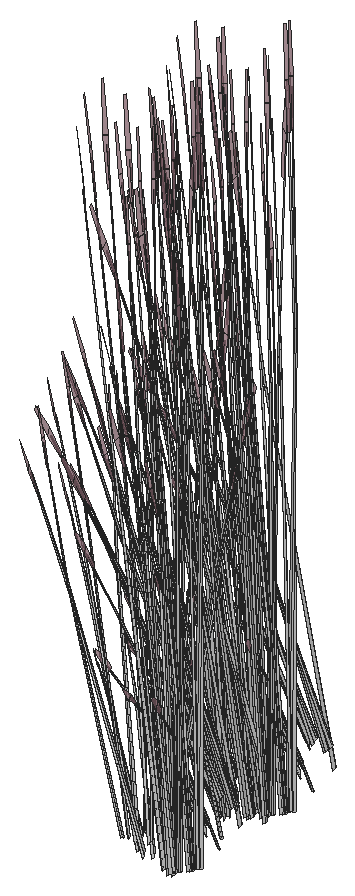
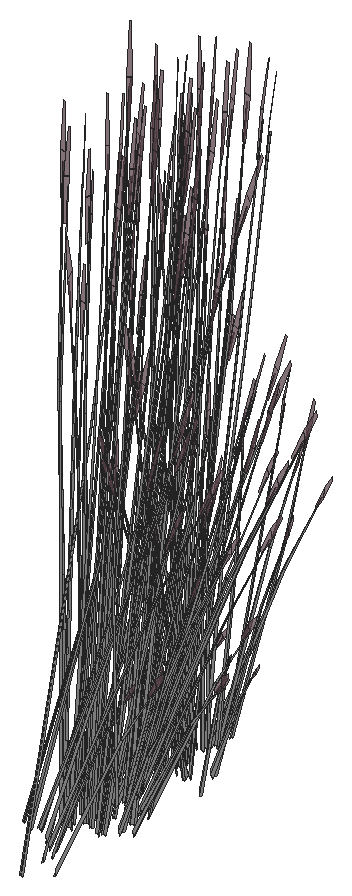
# SketchUp Ruby script. Lengths in inches.
U = 1.inch
M = Sketchup.active_model
def pt(a) = Geom::Point3d.new(a.map { |v| v * U })
def face(e, loops, mat)
  f = e.add_face(loops[0].map { |a| pt(a) })
  loops[1..].each { |l| e.add_face(l.map { |a| pt(a) }).erase! }
  f.material = f.back_material = mat if mat
  f
end
# faces: each face lists its corners as indices into pts; further lists are holes
def faces(e, pts, list, mat = nil) = list.each { |f| face(e, (f[0].is_a?(Array) ? f : [f]).map { |l| l.map { |i| pts[i] } }, mat) }
# xy, xz, yz: faces in a plane at the given z, y or x. An outline is a flat list of corners, or four numbers for a rectangle; further outlines are holes
def ring(l) = l.size == 4 ? [[l[0], l[1]], [l[2], l[1]], [l[2], l[3]], [l[0], l[3]]] : l.each_slice(2).to_a
def flat(e, list, mat, &to3) = list.each { |f| face(e, (f[0].is_a?(Array) ? f : [f]).map { |l| ring(l).map { |u, v| to3.(u, v) } }, mat) }
def xy(e, z, list, mat = nil) = flat(e, list, mat) { |x, y| [x, y, z] }
def xz(e, y, list, mat = nil) = flat(e, list, mat) { |x, z| [x, y, z] }
def yz(e, x, list, mat = nil) = flat(e, list, mat) { |y, z| [x, y, z] }
def lines(e, pts, list) = list.each { |a, b| e.add_line(pt(pts[a]), pt(pts[b])) }
# prism: a flat outline (further loops are holes) pulled along v
def prism(e, loops, v, mat = nil)
  f = face(e, loops, mat); d = Geom::Vector3d.new(v.map { |x| x * U })
  f.pushpull(f.normal.samedirection?(d) ? d.length : -d.length)
end
def box(e, o, s, mat = nil) = prism(e, [[o, [o[0] + s[0], o[1], o[2]], [o[0] + s[0], o[1] + s[1], o[2]], [o[0], o[1] + s[1], o[2]]]], [0, 0, s[2]], mat)
def at(x, y, z, deg = 0) = Geom::Transformation.translation(pt([x, y, z])) * Geom::Transformation.rotation(ORIGIN, Z_AXIS, deg.degrees)
def axes(o, x, y, z) = Geom::Transformation.new([*x, 0, *y, 0, *z, 0, *pt(o).to_a, 1])
def part(name) = M.definitions.add(name)
# library, detail: a bought-in or finely detailed component or shape, given as its bounding box
def library(name, o, s) = part(name).tap { |d| box(d.entities, o, s) }
def detail(e, o, s) = box(e.add_group.entities, o, s)
def put(e, d, t, mat = nil) = e.add_instance(d, t).tap { |i| i.material = mat if mat }
def group(e, t, mat = nil) = e.add_group.tap { |g| g.transformation = t; g.material = mat if mat }.entities
root = M.entities
M.materials.add("LightPink_Translucent").color = [144, 107, 117]
M.materials["LightPink_Translucent"].alpha = 0.75
M.materials.add("[_0053_Ivory_]").color = [200, 200, 200]
c1 = part("blade")
p = [[2.15,0.21,22],[0,0.17,0],[0.09,0.45,0],[2.18,0.31,22],[2.29,0.31,22],[0.38,0.45,0],
  [2.48,0.24,33],[2.49,0.24,33],[2.48,0.22,33]]
faces(c1.entities,p,[[0,1,2,3],[4,5,2,3],[6,3,4,7],[8,0,3,6]])
c2 = part("seeds")
p = [[0.3,-0.1,1.38],[-0.01,-0.03,1.59],[-0.01,-0.03,0.03],[0.14,-0.07,-0.07],[0.29,-0.03,3],[0.15,0.01,3.11]]
faces(c2.entities,p,[[0,1,2,3],[1,0,4,5]],"LightPink_Translucent")
c3 = part("blade with seeds")
put(c3.entities,c1,at(0,0,0))
put(c3.entities,c2,axes([2.4,0.25,30.99],[1.5799,-0.05474,1.17369],[-0.12525,1.92788,0.29478],[-0.07173,-0.02425,1.56792]))
put(root,c3,axes([629.08,303.62,255.53],[0.25192,-0.01424,1.71376],[-0.16712,0.61729,0.13857],[-0.35901,-0.03818,0.73262]),"[_0053_Ivory_]")
put(root,c3,axes([629.1875,294.41,255.53],[0.21074,-0.13302,1.71376],[0.17741,0.61464,0.13857],[-0.33083,0.13891,0.73262]),"[_0053_Ivory_]")
put(root,c3,axes([629.1875,304.71,255.53],[0.21074,-0.13302,1.71376],[0.17741,0.61464,0.13857],[-0.33083,0.13891,0.73262]),"[_0053_Ivory_]")
put(root,c3,axes([628.53,295.46,254.24],[0.21107,0.05162,1.43002],[0.13604,0.52729,-0.30754],[-0.28671,0.0987,0.61141]),"[_0053_Ivory_]")
put(root,c3,axes([628.53,305.75,254.24],[0.21107,0.05162,1.43002],[0.13604,0.52729,-0.30754],[-0.28671,0.0987,0.61141]),"[_0053_Ivory_]")
put(root,c3,axes([630.4,293.77,255],[0.17264,-0.09097,1.77064],[0.05953,0.63516,0.13857],[-0.37394,0.08428,0.63284]),"[_0053_Ivory_]")
put(root,c3,axes([630.4,304.0625,255],[0.17264,-0.09097,1.77064],[0.05953,0.63516,0.13857],[-0.37394,0.08428,0.63284]),"[_0053_Ivory_]")
put(root,c3,axes([629.83,303.05,256.63],[-0.60713,-0.01514,-0.71045],[0.04078,-0.63759,0.08574],[-0.25721,-0.06729,1.00501]),"[_0053_Ivory_]")
put(root,c3,axes([629.35,303.2,254.24],[0.11858,0.17508,1.43002],[-0.27325,0.4759,-0.30754],[-0.28057,-0.11375,0.61141]),"[_0053_Ivory_]")
put(root,c3,axes([628.86,293.85,256.18],[-0.50475,-0.17543,-0.35414],[0.14722,-0.5118,0.4572],[-0.20322,0.04693,0.87481]),"[_0053_Ivory_]")
put(root,c3,axes([628.86,304.15,256.18],[-0.50475,-0.17543,-0.35414],[0.14722,-0.5118,0.4572],[-0.20322,0.04693,0.87481]),"[_0053_Ivory_]")
put(root,c3,axes([629.56,302.63,255.53],[0.2256,0.10835,1.71376],[-0.46687,0.45453,0.13857],[-0.29098,-0.20505,0.73262]),"[_0053_Ivory_]")
put(root,c3,axes([629.56,313.02,255.53],[0.2256,0.10835,1.71376],[-0.46687,0.45453,0.13857],[-0.29098,-0.20505,0.73262]),"[_0053_Ivory_]")
put(root,c3,axes([629.21,294.12,256.33],[-0.16454,0.57202,-0.51099],[-0.56413,-0.19607,-0.3958],[-0.22713,0.05245,0.97773]),"[_0053_Ivory_]")
put(root,c3,axes([629.21,304.41,256.33],[-0.16454,0.57202,-0.51099],[-0.56413,-0.19607,-0.3958],[-0.22713,0.05245,0.97773]),"[_0053_Ivory_]")
put(root,c3,axes([629.63,303.17,256.33],[-0.44101,0.41656,-0.51099],[-0.38623,-0.44004,-0.3958],[-0.22407,-0.06338,0.97773]),"[_0053_Ivory_]")
put(root,c3,axes([628.92,304.375,253.15],[0.0154,0.09911,1.76342],[-0.31051,0.51756,-0.26939],[-0.22056,-0.02609,0.30037]),"[_0053_Ivory_]")
put(root,c3,axes([628.09,296.5625,254.42],[0.25312,-0.28501,1.1486],[0.09988,0.45119,0.84392],[-0.18292,0.08079,0.25299]),"[_0053_Ivory_]")
put(root,c3,axes([628.09,306.86,254.42],[0.25312,-0.28501,1.1486],[0.09988,0.45119,0.84392],[-0.18292,0.08079,0.25299]),"[_0053_Ivory_]")
put(root,c3,axes([629.47,302.78,256.18],[-0.34557,-0.39372,-0.35414],[0.39459,-0.37271,0.4572],[-0.20048,-0.05671,0.87481]),"[_0053_Ivory_]")
put(root,c3,axes([629.96,294.82,255.53],[0.1517,-0.19322,1.71376],[0.38303,0.52154,0.13857],[-0.26271,0.23751,0.73262]),"[_0053_Ivory_]")
put(root,c3,axes([629.96,305.12,255.53],[0.1517,-0.19322,1.71376],[0.38303,0.52154,0.13857],[-0.26271,0.23751,0.73262]),"[_0053_Ivory_]")
put(root,c3,axes([629.04,295.33,256.18],[-0.52868,0.08987,-0.35414],[-0.1396,-0.51376,0.4572],[-0.1515,0.13799,0.87481]),"[_0053_Ivory_]")
put(root,c3,axes([629.04,305.625,256.18],[-0.52868,0.08987,-0.35414],[-0.1396,-0.51376,0.4572],[-0.1515,0.13799,0.87481]),"[_0053_Ivory_]")
put(root,c3,axes([628.76,296.86,253.15],[0.08147,0.06283,1.76342],[0.13814,0.58211,-0.26939],[-0.18056,0.12413,0.30037]),"[_0053_Ivory_]")
put(root,c3,axes([628.64,303.73,254.42],[0.38775,-0.045,1.1486],[-0.24596,0.39648,0.84392],[-0.19161,-0.05948,0.25299]),"[_0053_Ivory_]")
put(root,c3,axes([629.84,295.3,255.53],[0.11309,-0.21615,1.71376],[0.47441,0.44731,0.13857],[-0.21402,0.27879,0.73262]),"[_0053_Ivory_]")
put(root,c3,axes([629.48,295.39,256.33],[0.15602,0.5742,-0.51099],[-0.59087,0.10045,-0.3958],[-0.16933,0.15423,0.97773]),"[_0053_Ivory_]")
put(root,c3,axes([629.48,305.69,256.33],[0.15602,0.5742,-0.51099],[-0.59087,0.10045,-0.3958],[-0.16933,0.15423,0.97773]),"[_0053_Ivory_]")
put(root,c3,axes([630.95,305.27,253.71],[-0.63179,-0.1031,-0.62353],[0.13332,-0.63596,-0.16365],[-0.18854,-0.07706,1.37633]),"[_0053_Ivory_]")
put(root,c3,axes([630.89,302.29,256.63],[-0.51789,-0.30395,-0.71045],[0.36805,-0.53263,0.08574],[-0.18764,-0.18149,1.00501]),"[_0053_Ivory_]")
put(root,c3,axes([630.89,312.68,256.63],[-0.51789,-0.30395,-0.71045],[0.36805,-0.53263,0.08574],[-0.18764,-0.18149,1.00501]),"[_0053_Ivory_]")
put(root,c3,axes([630.65,302.31,256.33],[-0.59932,0.14948,-0.51099],[-0.10484,-0.56611,-0.3958],[-0.16097,-0.16223,0.97773]),"[_0053_Ivory_]")
put(root,c3,axes([630.125,306.48,253.67],[-0.56842,-0.31443,-0.49651],[0.33976,-0.56381,0],[-0.12946,-0.07161,1.57504]),"[_0053_Ivory_]")
put(root,c3,axes([629.875,301.79,253.15],[-0.05883,0.08284,1.76342],[-0.59454,0.17861,-0.26939],[-0.14363,-0.16248,0.30037]),"[_0053_Ivory_]")
put(root,c3,axes([629.875,312.18,253.15],[-0.05883,0.08284,1.76342],[-0.59454,0.17861,-0.26939],[-0.14363,-0.16248,0.30037]),"[_0053_Ivory_]")
put(root,c3,axes([630.47,296.5625,254.03],[-0.37973,0.63014,0],[-0.6353,-0.35142,-0.51607],[-0.14469,-0.08004,1.63711]),"[_0053_Ivory_]")
put(root,c3,axes([630.47,306.86,254.03],[-0.37973,0.63014,0],[-0.6353,-0.35142,-0.51607],[-0.14469,-0.08004,1.63711]),"[_0053_Ivory_]")
put(root,c3,axes([629.78,297.47,254.24],[0.19166,-0.0992,1.43002],[0.4732,0.29912,-0.30754],[-0.14084,0.25882,0.61141]),"[_0053_Ivory_]")
put(root,c3,axes([629.51,302.11,253.78],[-0.1752,0.51349,-0.03893],[-0.53924,-0.15795,-0.17649],[-0.08187,-0.08399,0.58215]),"[_0053_Ivory_]")
put(root,c3,axes([630.3125,301.47,254.24],[-0.03678,0.20572,1.43002],[-0.53767,0.17221,-0.30754],[-0.12568,-0.26589,0.61141]),"[_0053_Ivory_]")
put(root,c3,axes([630.3125,311.86,254.24],[-0.03678,0.20572,1.43002],[-0.53767,0.17221,-0.30754],[-0.12568,-0.26589,0.61141]),"[_0053_Ivory_]")
put(root,c3,axes([630.49,302,255.53],[0.13883,0.2019,1.71376],[-0.64153,0.16998,0.13857],[-0.14499,-0.31697,0.73262]),"[_0053_Ivory_]")
put(root,c3,axes([630.49,312.39,255.53],[0.13883,0.2019,1.71376],[-0.64153,0.16998,0.13857],[-0.14499,-0.31697,0.73262]),"[_0053_Ivory_]")
put(root,c3,axes([631.67,295.07,254.32],[-0.61322,0.4175,-0.29095],[-0.40778,-0.58992,-0.50002],[-0.1513,-0.05991,1.59708]),"[_0053_Ivory_]")
put(root,c3,axes([631.67,305.37,254.32],[-0.61322,0.4175,-0.29095],[-0.40778,-0.58992,-0.50002],[-0.1513,-0.05991,1.59708]),"[_0053_Ivory_]")
put(root,c3,axes([630.71,301.89,256.18],[-0.0938,-0.50652,-0.35414],[0.53623,-0.13375,0.4572],[-0.14403,-0.14515,0.87481]),"[_0053_Ivory_]")
put(root,c3,axes([630.71,312.28,256.18],[-0.0938,-0.50652,-0.35414],[0.53623,-0.13375,0.4572],[-0.14403,-0.14515,0.87481]),"[_0053_Ivory_]")
put(root,c3,axes([629.22,304.46,254.03],[-0.75945,0,0],[0,-0.70283,-0.51607],[0,-0.16007,1.63711]),"[_0053_Ivory_]")
put(root,c3,axes([630.28,306.24,253.68],[-0.14267,-0.54795,-0.30978],[0.56663,-0.1556,0.30978],[-0.11423,-0.06319,1.38974]),"[_0053_Ivory_]")
put(root,c3,axes([629.97,296.52,256.18],[-0.41095,0.33109,-0.35414],[-0.38901,-0.37805,0.4572],[-0.05919,0.19208,0.87481]),"[_0053_Ivory_]")
put(root,c3,axes([632.08,295.53,253.71],[-0.40909,0.47266,-0.62353],[-0.50819,-0.4286,-0.16365],[-0.16393,0.11791,1.37633]),"[_0053_Ivory_]")
put(root,c3,axes([632.08,305.82,253.71],[-0.40909,0.47266,-0.62353],[-0.50819,-0.4286,-0.16365],[-0.16393,0.11791,1.37633]),"[_0053_Ivory_]")
put(root,c3,axes([629.8,304.27,253.98],[-0.56493,0.5287,0.30756],[-0.56528,-0.52313,-0.36492],[-0.01973,-0.15014,1.64885]),"[_0053_Ivory_]")
put(root,c3,axes([632.13,305.73,254.98],[0.52485,0.25358,1.51261],[-0.51417,0.54629,0.59816],[-0.23031,-0.32378,1.26806]),"[_0053_Ivory_]")
put(root,c3,axes([630.125,301.13,254.42],[0.31682,0.21887,1.1486],[-0.4614,0.13157,0.84392],[-0.09872,-0.16821,0.25299]),"[_0053_Ivory_]")
put(root,c3,axes([630.125,311.52,254.42],[0.31682,0.21887,1.1486],[-0.4614,0.13157,0.84392],[-0.09872,-0.16821,0.25299]),"[_0053_Ivory_]")
put(root,c3,axes([632.36,295.26,254.12],[-0.59306,-0.50614,-0.25192],[0.49904,-0.56836,0.5513],[-0.1597,0.05921,1.68216]),"[_0053_Ivory_]")
put(root,c3,axes([632.36,305.56,254.12],[-0.59306,-0.50614,-0.25192],[0.49904,-0.56836,0.5513],[-0.1597,0.05921,1.68216]),"[_0053_Ivory_]")
put(root,c3,axes([631.28,305.07,253.86],[-0.36485,-0.52782,-0.44739],[0.55265,-0.37168,0.21531],[-0.11807,-0.06531,1.43643]),"[_0053_Ivory_]")
put(root,c3,axes([630.25,296.17,256.99],[-0.0158,0.58168,-0.7886],[-0.66548,-0.03907,0.09517],[-0.07023,0.24643,1.11556]),"[_0053_Ivory_]")
put(root,c3,axes([630.24,297.81,254.42],[-0.01572,-0.37392,1.1486],[0.39276,0.26669,0.84392],[-0.07724,0.17822,0.25299]),"[_0053_Ivory_]")
put(root,c3,axes([632.06,295.15,253.86],[-0.65953,0.03882,-0.44739],[-0.05964,-0.64439,0.21531],[-0.11807,0.06531,1.43643]),"[_0053_Ivory_]")
put(root,c3,axes([632.06,305.45,253.86],[-0.65953,0.03882,-0.44739],[-0.05964,-0.64439,0.21531],[-0.11807,0.06531,1.43643]),"[_0053_Ivory_]")
put(root,c3,axes([630.8,296.23,254.13],[0.56842,0.31443,0.49651],[-0.33976,0.56381,0],[-0.12946,-0.07161,1.57504]),"[_0053_Ivory_]")
put(root,c3,axes([630.8,306.53,254.13],[0.56842,0.31443,0.49651],[-0.33976,0.56381,0],[-0.12946,-0.07161,1.57504]),"[_0053_Ivory_]")
put(root,c3,axes([630.03,296.99,255.02],[0.01334,-0.32463,1.54345],[0.60018,0.17147,0.21329],[-0.052,0.34598,0.72882]),"[_0053_Ivory_]")
put(root,c3,axes([631.33,305.375,254.09],[0.16098,-0.74515,-0.23429],[0.76326,0.12989,0.51271],[-0.13337,-0.1029,1.5644]),"[_0053_Ivory_]")
put(root,c3,axes([631.61,295.25,254.27],[-0.11717,0.56122,0.1448],[-0.57245,-0.09742,-0.41347],[-0.10418,-0.05763,1.26744]),"[_0053_Ivory_]")
put(root,c3,axes([631.61,305.55,254.27],[-0.11717,0.56122,0.1448],[-0.57245,-0.09742,-0.41347],[-0.10418,-0.05763,1.26744]),"[_0053_Ivory_]")
put(root,c3,axes([632.75,296.82,253.67],[-0.56842,0.31443,-0.49651],[-0.33976,-0.56381,0],[-0.12946,0.07161,1.57504]),"[_0053_Ivory_]")
put(root,c3,axes([632.75,307.11,253.67],[-0.56842,0.31443,-0.49651],[-0.33976,-0.56381,0],[-0.12946,0.07161,1.57504]),"[_0053_Ivory_]")
put(root,c3,axes([629.39,303.98,253.67],[0,-0.62885,-0.49651],[0.67951,0,0],[0,-0.14322,1.57504]),"[_0053_Ivory_]")
put(root,c3,axes([629.68,304.5625,254.13],[0,0.62885,0.49651],[-0.67951,0,0],[0,-0.14322,1.57504]),"[_0053_Ivory_]")
put(root,c3,axes([632.79,296.65,253.85],[-0.37499,-0.63235,-0.05142],[0.6353,-0.35142,0.51607],[-0.15655,0.0602,1.6363]),"[_0053_Ivory_]")
put(root,c3,axes([632.79,306.94,253.85],[-0.37499,-0.63235,-0.05142],[0.6353,-0.35142,0.51607],[-0.15655,0.0602,1.6363]),"[_0053_Ivory_]")
put(root,c3,axes([630.38,296.36,256.66],[0.43478,0.42253,-0.5672],[-0.45929,0.37004,-0.43934],[-0.06615,0.21468,1.08528]),"[_0053_Ivory_]")
put(root,c3,axes([632.62,296.57,253.68],[-0.56663,-0.1556,-0.30978],[0.14267,-0.54795,0.30978],[-0.11423,0.06319,1.38974]),"[_0053_Ivory_]")
put(root,c3,axes([632.62,306.86,253.68],[-0.56663,-0.1556,-0.30978],[0.14267,-0.54795,0.30978],[-0.11423,0.06319,1.38974]),"[_0053_Ivory_]")
put(root,c3,axes([631.16,304.71,254.32],[-0.68399,-0.30005,-0.29095],[0.32934,-0.63331,-0.50002],[-0.0215,-0.15549,1.59708]),"[_0053_Ivory_]")
put(root,c3,axes([632.94,294.23,254.5],[-0.01659,-0.59209,1.41272],[0.75089,0.15348,0.59816],[-0.1776,0.32398,1.3335]),"[_0053_Ivory_]")
put(root,c3,axes([632.94,304.52,254.5],[-0.01659,-0.59209,1.41272],[0.75089,0.15348,0.59816],[-0.1776,0.32398,1.3335]),"[_0053_Ivory_]")
put(root,c3,axes([629.91,297,254.48],[0.55175,-0.11136,0.06507],[0.12684,0.44864,-0.86304],[-0.03498,0.22711,0.7736]),"[_0053_Ivory_]")
put(root,c3,axes([632.52,294.98,254.32],[0.07077,0.71755,-0.29095],[-0.73712,0.04339,-0.50002],[-0.1298,0.09558,1.59708]),"[_0053_Ivory_]")
put(root,c3,axes([632.52,305.28,254.32],[0.07077,0.71755,-0.29095],[-0.73712,0.04339,-0.50002],[-0.1298,0.09558,1.59708]),"[_0053_Ivory_]")
put(root,c3,axes([630.86,304.07,253.75],[-0.24943,-0.64486,-0.69835],[0.71849,-0.23224,-0.18329],[-0.02757,-0.21836,1.54149]),"[_0053_Ivory_]")
put(root,c3,axes([630.86,314.46,253.75],[-0.24943,-0.64486,-0.69835],[0.71849,-0.23224,-0.18329],[-0.02757,-0.21836,1.54149]),"[_0053_Ivory_]")
put(root,c3,axes([631.98,302.05,256.33],[-0.59704,-0.15764,-0.51099],[0.20464,-0.54049,-0.3958],[-0.05475,-0.21761,0.97773]),"[_0053_Ivory_]")
put(root,c3,axes([631.98,312.4375,256.33],[-0.59704,-0.15764,-0.51099],[0.20464,-0.54049,-0.3958],[-0.05475,-0.21761,0.97773]),"[_0053_Ivory_]")
put(root,c3,axes([630.88,295.76,255.53],[-0.01487,-0.24136,1.71376],[0.64429,0.16012,0.13857],[-0.03985,0.34396,0.73262]),"[_0053_Ivory_]")
put(root,c3,axes([629.68,303.99,253.68],[0.42396,-0.39235,-0.30978],[0.42396,0.39235,0.30978],[0,-0.12637,1.38974]),"[_0053_Ivory_]")
put(root,c3,axes([631.59,301.46,253.78],[-0.4197,0.36076,-0.03893],[-0.38456,-0.39511,-0.17649],[-0.02707,-0.11196,0.58215]),"[_0053_Ivory_]")
put(root,c3,axes([631.42,305.01,254.01],[0.76764,0.13249,0.45755],[-0.15622,0.74829,0.17955],[-0.11218,-0.07226,1.58856]),"[_0053_Ivory_]")
put(root,c3,axes([631.22,304.88,254.37],[-0.29468,0.56664,0.44739],[-0.61229,-0.27271,-0.21531],[0,-0.13062,1.43643]),"[_0053_Ivory_]")
put(root,c3,axes([632.2,302.15,256.63],[-0.28988,-0.51132,-0.71045],[0.59671,-0.28496,0.08574],[-0.06778,-0.24706,1.00501]),"[_0053_Ivory_]")
put(root,c3,axes([632.2,312.54,256.63],[-0.28988,-0.51132,-0.71045],[0.59671,-0.28496,0.08574],[-0.06778,-0.24706,1.00501]),"[_0053_Ivory_]")
put(root,c3,axes([631.01,306.21,254.13],[0.65264,-0.16691,0.17642],[0.16115,0.62115,0.35086],[-0.05821,-0.0905,1.60407]),"[_0053_Ivory_]")
put(root,c3,axes([631.85,296.01,253.85],[-0.61229,-0.28233,0],[0.29468,-0.58663,0],[0,0,1.62707]),"[_0053_Ivory_]")
put(root,c3,axes([631.85,306.31,253.85],[-0.61229,-0.28233,0],[0.29468,-0.58663,0],[0,0,1.62707]),"[_0053_Ivory_]")
put(root,c3,axes([633.27,296.72,254.03],[0.37973,0.63014,0],[-0.6353,0.35142,-0.51607],[-0.14469,0.08004,1.63711]),"[_0053_Ivory_]")
put(root,c3,axes([633.27,307.02,254.03],[0.37973,0.63014,0],[-0.6353,0.35142,-0.51607],[-0.14469,0.08004,1.63711]),"[_0053_Ivory_]")
put(root,c3,axes([632.95,295.95,254.13],[0.17545,-0.62497,0.17642],[0.64204,0.17686,0.35086],[-0.11091,0.00304,1.60407]),"[_0053_Ivory_]")
put(root,c3,axes([632.95,306.24,254.13],[0.17545,-0.62497,0.17642],[0.64204,0.17686,0.35086],[-0.11091,0.00304,1.60407]),"[_0053_Ivory_]")
put(root,c3,axes([632.66,295.12,254.27],[0.44871,0.37783,0.1448],[-0.37428,0.42627,-0.41347],[-0.10418,0.05763,1.26744]),"[_0053_Ivory_]")
put(root,c3,axes([632.66,305.41,254.27],[0.44871,0.37783,0.1448],[-0.37428,0.42627,-0.41347],[-0.10418,0.05763,1.26744]),"[_0053_Ivory_]")
put(root,c3,axes([632.5,304.95,253.95],[-0.56493,-0.54126,-0.06131],[0.56528,-0.54159,0],[-0.01973,-0.0189,1.75571]),"[_0053_Ivory_]")
put(root,c3,axes([632.65,294.84,254.37],[0.65953,-0.03882,0.44739],[0.05964,0.64439,-0.21531],[-0.11807,0.06531,1.43643]),"[_0053_Ivory_]")
put(root,c3,axes([632.65,305.14,254.37],[0.65953,-0.03882,0.44739],[0.05964,0.64439,-0.21531],[-0.11807,0.06531,1.43643]),"[_0053_Ivory_]")
put(root,c3,axes([632.81,296.32,253.98],[0.76036,0.2044,0.30756],[-0.19023,0.7306,-0.36492],[-0.12585,0.09144,1.64885]),"[_0053_Ivory_]")
put(root,c3,axes([632.81,306.62,253.98],[0.76036,0.2044,0.30756],[-0.19023,0.7306,-0.36492],[-0.12585,0.09144,1.64885]),"[_0053_Ivory_]")
put(root,c3,axes([631.7,301.01,253.15],[-0.10187,0.02266,1.76342],[-0.56336,-0.25503,-0.26939],[0.00945,-0.21273,0.30037]),"[_0053_Ivory_]")
put(root,c3,axes([631.7,311.4,253.15],[-0.10187,0.02266,1.76342],[-0.56336,-0.25503,-0.26939],[0.00945,-0.21273,0.30037]),"[_0053_Ivory_]")
put(root,c3,axes([633.13,296.28,254.13],[0.56842,-0.31443,0.49651],[0.33976,0.56381,0],[-0.12946,0.07161,1.57504]),"[_0053_Ivory_]")
put(root,c3,axes([633.13,306.58,254.13],[0.56842,-0.31443,0.49651],[0.33976,0.56381,0],[-0.12946,0.07161,1.57504]),"[_0053_Ivory_]")
put(root,c3,axes([632.25,301.71,256.18],[0.1831,-0.48359,-0.35414],[0.53419,0.14105,0.4572],[-0.04898,-0.1947,0.87481]),"[_0053_Ivory_]")
